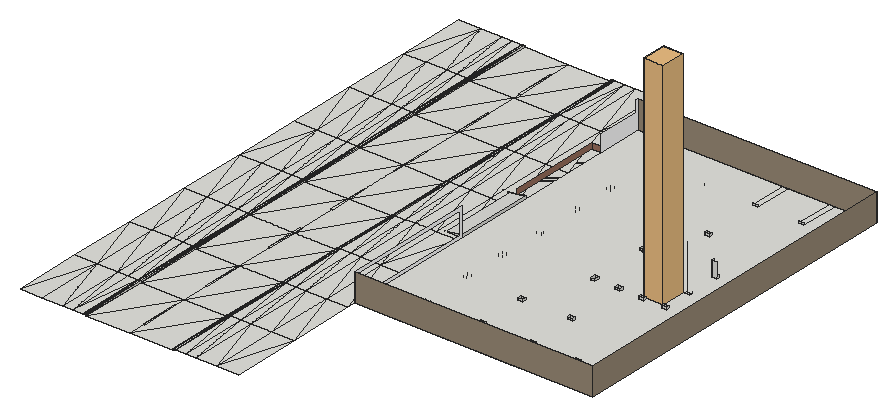
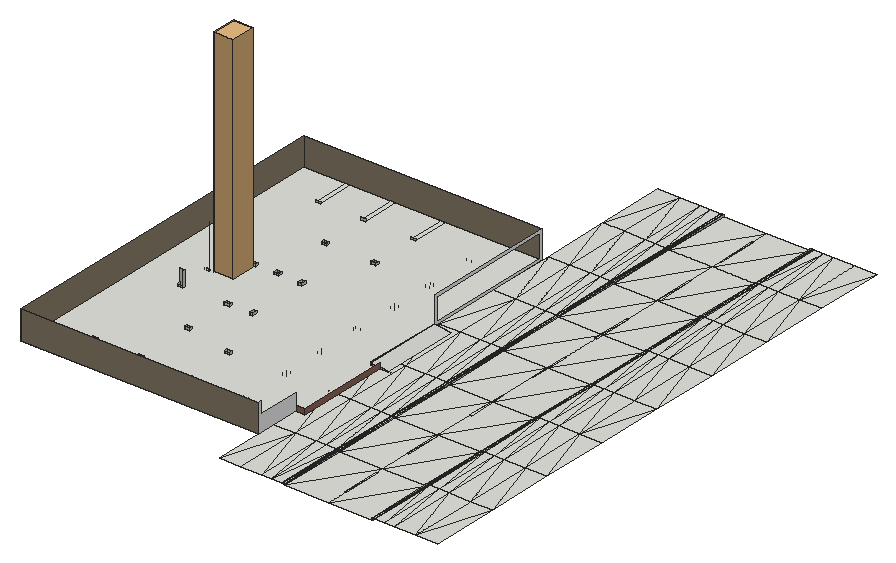
# SketchUp Ruby script. Lengths in inches.
U = 1.inch
M = Sketchup.active_model
def pt(a) = Geom::Point3d.new(a.map { |v| v * U })
def face(e, loops, mat)
  f = e.add_face(loops[0].map { |a| pt(a) })
  loops[1..].each { |l| e.add_face(l.map { |a| pt(a) }).erase! }
  f.material = f.back_material = mat if mat
  f
end
# faces: each face lists its corners as indices into pts; further lists are holes
def faces(e, pts, list, mat = nil) = list.each { |f| face(e, (f[0].is_a?(Array) ? f : [f]).map { |l| l.map { |i| pts[i] } }, mat) }
# xy, xz, yz: faces in a plane at the given z, y or x. An outline is a flat list of corners, or four numbers for a rectangle; further outlines are holes
def ring(l) = l.size == 4 ? [[l[0], l[1]], [l[2], l[1]], [l[2], l[3]], [l[0], l[3]]] : l.each_slice(2).to_a
def flat(e, list, mat, &to3) = list.each { |f| face(e, (f[0].is_a?(Array) ? f : [f]).map { |l| ring(l).map { |u, v| to3.(u, v) } }, mat) }
def xy(e, z, list, mat = nil) = flat(e, list, mat) { |x, y| [x, y, z] }
def xz(e, y, list, mat = nil) = flat(e, list, mat) { |x, z| [x, y, z] }
def yz(e, x, list, mat = nil) = flat(e, list, mat) { |y, z| [x, y, z] }
def lines(e, pts, list) = list.each { |a, b| e.add_line(pt(pts[a]), pt(pts[b])) }
# prism: a flat outline (further loops are holes) pulled along v
def prism(e, loops, v, mat = nil)
  f = face(e, loops, mat); d = Geom::Vector3d.new(v.map { |x| x * U })
  f.pushpull(f.normal.samedirection?(d) ? d.length : -d.length)
end
def box(e, o, s, mat = nil) = prism(e, [[o, [o[0] + s[0], o[1], o[2]], [o[0] + s[0], o[1] + s[1], o[2]], [o[0], o[1] + s[1], o[2]]]], [0, 0, s[2]], mat)
def at(x, y, z, deg = 0) = Geom::Transformation.translation(pt([x, y, z])) * Geom::Transformation.rotation(ORIGIN, Z_AXIS, deg.degrees)
def axes(o, x, y, z) = Geom::Transformation.new([*x, 0, *y, 0, *z, 0, *pt(o).to_a, 1])
def part(name) = M.definitions.add(name)
# library, detail: a bought-in or finely detailed component or shape, given as its bounding box
def library(name, o, s) = part(name).tap { |d| box(d.entities, o, s) }
def detail(e, o, s) = box(e.add_group.entities, o, s)
def put(e, d, t, mat = nil) = e.add_instance(d, t).tap { |i| i.material = mat if mat }
def group(e, t, mat = nil) = e.add_group.tap { |g| g.transformation = t; g.material = mat if mat }.entities
root = M.entities
M.materials.add("Bricks Weathered E01 100cm\#1").color = [154, 112, 93]
M.materials.add("Paint Brown Gloss 1.5cm").color = [255, 255, 255]
M.materials.add("Paint Brown Gloss 1.5cm\#1").color = [255, 255, 255]
M.materials.add("Wall Paint Bumpy 01 Ochre 100cm").color = [152, 138, 118]
c1 = library("Untitled",[11.72,11.72,0],[78.74,90.55,365.17])
xy(root,-10.11,[[1303.23,0,1424.89,0,1424.89,191.1],[1303.23,0,1424.89,191.1,1303.23,191.1],[1424.89,0,1546.54,0,1546.54,191.1],[1424.89,0,1546.54,191.1,1424.89,191.1],[1303.23,191.1,1424.89,191.1,1424.89,382.19],
  [1303.23,191.1,1424.89,382.19,1303.23,382.19],[1424.89,191.1,1546.54,191.1,1546.54,382.19],[1424.89,191.1,1546.54,382.19,1424.89,382.19],[1303.23,382.19,1424.89,382.19,1424.89,573.29],[1303.23,382.19,1424.89,573.29,1303.23,573.29],
  [1424.89,382.19,1546.54,382.19,1546.54,573.29],[1424.89,382.19,1546.54,573.29,1424.89,573.29],[1303.23,573.29,1424.89,573.29,1424.89,764.38],[1303.23,573.29,1424.89,764.38,1303.23,764.38],[1424.89,573.29,1546.54,573.29,1546.54,764.38],
  [1424.89,573.29,1546.54,764.38,1424.89,764.38],[1303.23,764.38,1424.89,764.38,1424.89,955.48],[1303.23,764.38,1424.89,955.48,1303.23,955.48],[1424.89,764.38,1546.54,764.38,1546.54,955.48],[1424.89,764.38,1546.54,955.48,1424.89,955.48],
  [1303.23,955.48,1424.89,1146.57,1303.23,1146.57],[1303.23,955.48,1424.89,955.48,1424.89,1146.57],[1424.89,955.48,1546.54,1146.57,1424.89,1146.57],[1424.89,955.48,1546.54,955.48,1546.54,1146.57],[1303.23,1146.57,1424.89,1146.57,1424.89,1337.67],
  [1303.23,1146.57,1424.89,1337.67,1303.23,1337.67],[1424.89,1146.57,1546.54,1146.57,1546.54,1337.67],[1424.89,1146.57,1546.54,1337.67,1424.89,1337.67],[1303.23,1337.67,1424.89,1337.67,1424.89,1528.76],[1303.23,1337.67,1424.89,1528.76,1303.23,1528.76],
  [1424.89,1337.67,1546.54,1337.67,1546.54,1528.76],[1424.89,1337.67,1546.54,1528.76,1424.89,1528.76]])
xy(root,-10.1,[[1422.83,51.125,1426.94,160.2,1422.83,160.2],[1422.83,51.125,1426.94,51.125,1426.94,160.2],[1422.83,269.27,1426.94,269.27,1426.94,378.35],[1422.83,269.27,1426.94,378.35,1422.83,378.35],[1422.83,487.42,1426.94,487.42,1426.94,596.5],
  [1422.83,487.42,1426.94,596.5,1422.83,596.5],[1422.83,705.57,1426.94,705.57,1426.94,814.64],[1422.83,705.57,1426.94,814.64,1422.83,814.64],[1422.83,923.72,1426.94,1032.79,1422.83,1032.79],[1422.83,923.72,1426.94,923.72,1426.94,1032.79],
  [1422.83,1141.87,1426.94,1141.87,1426.94,1250.94],[1422.83,1141.87,1426.94,1250.94,1422.83,1250.94],[1422.83,1360.02,1426.94,1360.02,1426.94,1469.09],[1422.83,1360.02,1426.94,1469.09,1422.83,1469.09]])
xy(root,-6,[[1296.67,0,1297.07,0,1297.07,0.65],[1296.67,0,1297.07,0.65,1296.67,0.65],[1297.07,0,1302.39,0,1302.39,0.65],[1297.07,0,1302.39,0.65,1297.07,0.65],[1302.39,0,1302.75,0,1302.75,0.65],
  [1302.39,0,1302.75,0.65,1302.39,0.65],[1547.03,0,1547.61,0,1547.61,0.61],[1547.03,0,1547.61,0.61,1547.03,0.61],[1547.61,0,1552.83,0,1552.83,0.61],[1547.61,0,1552.83,0.61,1547.61,0.61],
  [1552.83,0,1553.1,0,1553.1,0.61],[1552.83,0,1553.1,0.61,1552.83,0.61],[1553.68,0,1554.02,0,1554.02,191.1],[1553.68,0,1554.02,191.1,1553.68,191.1],[1554.02,0,1582.4375,0,1554.02,191.1],
  [1582.4375,0,1582.4375,191.1,1554.02,191.1],[1582.4375,0,1610.85,0,1582.4375,191.1],[1610.85,0,1610.85,191.1,1582.4375,191.1],[1610.85,0,1668.2,0,1610.85,191.1],[1668.2,0,1668.2,191.1,1610.85,191.1],
  [1668.2,0,1729.02,0,1729.02,191.09],[1668.2,0,1729.02,191.09,1668.2,191.1],[1120.75,0.01,1181.58,0.01,1181.58,191.1],[1120.75,0.01,1181.58,191.1,1120.75,191.1],[1181.58,0.01,1238.93,0.01,1181.58,191.1],
  [1238.93,0.01,1238.93,191.1,1181.58,191.1],[1238.93,0.01,1267.34,0.01,1238.93,191.1],[1267.34,0.01,1267.34,191.1,1238.93,191.1],[1267.34,0.01,1295.75,0.01,1295.75,191.1],[1267.34,0.01,1295.75,191.1,1267.34,191.1],
  [1295.75,0.01,1296.1,0.01,1296.1,191.1],[1295.75,0.01,1296.1,191.1,1295.75,191.1],[1547.03,0.61,1547.61,0.61,1547.61,191.1],[1547.03,0.61,1547.61,191.1,1547.03,191.1],[1547.61,0.61,1552.83,0.61,1552.83,191.1],
  [1547.61,0.61,1552.83,191.1,1547.61,191.1],[1552.83,0.61,1553.1,0.61,1553.1,191.1],[1552.83,0.61,1553.1,191.1,1552.83,191.1],[1296.67,0.65,1297.07,0.65,1297.07,191.1],[1296.67,0.65,1297.07,191.1,1296.67,191.1],
  [1297.07,0.65,1302.39,0.65,1302.39,191.1],[1297.07,0.65,1302.39,191.1,1297.07,191.1],[1302.39,0.65,1302.75,0.65,1302.75,191.1],[1302.39,0.65,1302.75,191.1,1302.39,191.1],[1729.02,191.09,1668.2,382.19,1668.2,191.1],
  [1729.02,191.09,1729.02,382.19,1668.2,382.19],[1120.75,191.1,1181.58,191.1,1120.75,382.2],[1181.58,191.1,1181.58,382.2,1120.75,382.2],[1181.58,191.1,1238.93,191.1,1181.58,382.2],[1238.93,191.1,1238.93,382.2,1181.58,382.2],
  [1238.93,191.1,1267.34,191.1,1238.93,382.2],[1267.34,191.1,1267.34,382.2,1238.93,382.2],[1267.34,191.1,1295.75,191.1,1267.34,382.2],[1295.75,191.1,1295.75,382.2,1267.34,382.2],[1295.75,191.1,1296.1,191.1,1296.1,382.2],
  [1295.75,191.1,1296.1,382.2,1295.75,382.2],[1296.67,191.1,1297.07,191.1,1297.07,382.19],[1296.67,191.1,1297.07,382.19,1296.67,382.19],[1297.07,191.1,1302.39,191.1,1297.07,382.19],[1302.39,191.1,1302.39,382.19,1297.07,382.19],
  [1302.39,191.1,1302.75,191.1,1302.39,382.19],[1302.75,191.1,1302.75,382.19,1302.39,382.19],[1547.03,191.1,1547.61,191.1,1547.61,382.19],[1547.03,191.1,1547.61,382.19,1547.03,382.19],[1547.61,191.1,1552.83,191.1,1547.61,382.19],
  [1552.83,191.1,1552.83,382.19,1547.61,382.19],[1552.83,191.1,1553.1,191.1,1552.83,382.19],[1553.1,191.1,1553.1,382.19,1552.83,382.19],[1553.68,191.1,1554.02,191.1,1554.02,382.19],[1553.68,191.1,1554.02,382.19,1553.68,382.19],
  [1554.02,191.1,1582.4375,191.1,1554.02,382.19],[1582.4375,191.1,1582.4375,382.19,1554.02,382.19],[1582.4375,191.1,1610.85,191.1,1582.4375,382.19],[1610.85,191.1,1610.85,382.19,1582.4375,382.19],[1610.85,191.1,1668.2,191.1,1610.85,382.19],
  [1668.2,191.1,1668.2,382.19,1610.85,382.19],[1296.67,382.19,1297.07,382.19,1297.07,573.29],[1296.67,382.19,1297.07,573.29,1296.67,573.29],[1297.07,382.19,1302.39,382.19,1297.07,573.29],[1302.39,382.19,1302.39,573.29,1297.07,573.29],
  [1302.39,382.19,1302.75,382.19,1302.39,573.29],[1302.75,382.19,1302.75,573.29,1302.39,573.29],[1547.03,382.19,1547.61,382.19,1547.61,573.29],[1547.03,382.19,1547.61,573.29,1547.03,573.29],[1547.61,382.19,1552.83,382.19,1547.61,573.29],
  [1552.83,382.19,1552.83,573.29,1547.61,573.29],[1552.83,382.19,1553.1,382.19,1552.83,573.29],[1553.1,382.19,1553.1,573.29,1552.83,573.29],[1553.68,382.19,1554.02,382.19,1554.02,573.29],[1553.68,382.19,1554.02,573.29,1553.68,573.29],
  [1554.02,382.19,1582.4375,382.19,1554.02,573.29],[1582.4375,382.19,1582.4375,573.29,1554.02,573.29],[1582.4375,382.19,1610.85,382.19,1582.4375,573.29],[1610.85,382.19,1610.85,573.29,1582.4375,573.29],[1610.85,382.19,1668.2,382.19,1610.85,573.29],
  [1668.2,382.19,1668.2,573.29,1610.85,573.29],[1668.2,382.19,1729.02,382.19,1668.2,573.29],[1729.02,382.19,1729.02,573.29,1668.2,573.29],[1120.75,382.2,1181.58,382.2,1120.75,573.29],[1181.58,382.2,1181.58,573.29,1120.75,573.29],
  [1181.58,382.2,1238.93,382.2,1181.58,573.29],[1238.93,382.2,1238.93,573.29,1181.58,573.29],[1238.93,382.2,1267.34,382.2,1238.93,573.29],[1267.34,382.2,1267.34,573.29,1238.93,573.29],[1267.34,382.2,1295.75,382.2,1267.34,573.29],
  [1295.75,382.2,1295.75,573.29,1267.34,573.29],[1295.75,382.2,1296.1,382.2,1296.1,573.29],[1295.75,382.2,1296.1,573.29,1295.75,573.29],[[1729.02,404.67,1729.02,1000.17,1704.32,1000.17,1704.32,1262.67,1729.02,1262.67,1729.02,1391.67,2132.52,1391.67,2132.52,1286.67,2146.52,1286.67,2146.52,1391.67,2262.52,1391.67,2262.52,1286.67,2276.52,1286.67,2276.52,1391.67,2393.52,1391.67,2393.52,404.67,2276.52,404.67,2276.52,509.67,2262.52,509.67,2262.52,404.67,2149.52,404.67,2149.52,509.67,2135.52,509.67,2135.52,404.67,2011.02,404.67,2011.02,509.67,1997.02,509.67,1997.02,404.67],[2132.52,980.67,2146.52,989.67],[2262.52,980.67,2276.52,989.67],[2262.52,806.67,2276.52,815.67],[2066.52,806.67,2075.52,820.67],[1997.02,1148.67,2011.02,1157.67],[2132.52,1118.67,2146.52,1127.67],[2066.52,975.67,2075.52,989.67],[2262.52,887.67,2276.52,896.67],[2132.52,806.67,2146.52,815.67],[1997.02,638.67,2011.02,647.67],[2198.52,806.67,2212.52,815.67],[2135.52,638.67,2149.52,647.67]],[1997.02,404.67,2011.02,509.67],
  [2135.52,404.67,2149.52,509.67],[2262.52,404.67,2276.52,509.67],[1120.75,573.29,1181.58,573.29,1120.75,764.39],[1181.58,573.29,1181.58,764.39,1120.75,764.39],[1181.58,573.29,1238.93,573.29,1181.58,764.39],
  [1238.93,573.29,1238.93,764.39,1181.58,764.39],[1238.93,573.29,1267.34,573.29,1238.93,764.39],[1267.34,573.29,1267.34,764.39,1238.93,764.39],[1267.34,573.29,1295.75,573.29,1267.34,764.39],[1295.75,573.29,1295.75,764.39,1267.34,764.39],
  [1295.75,573.29,1296.1,573.29,1296.1,764.39],[1295.75,573.29,1296.1,764.39,1295.75,764.39],[1296.67,573.29,1297.07,573.29,1296.67,764.38],[1297.07,573.29,1297.07,764.38,1296.67,764.38],[1297.07,573.29,1302.39,573.29,1297.07,764.38],
  [1302.39,573.29,1302.39,764.38,1297.07,764.38],[1302.39,573.29,1302.75,573.29,1302.75,764.38],[1302.39,573.29,1302.75,764.38,1302.39,764.38],[1547.03,573.29,1547.61,573.29,1547.03,764.38],[1547.61,573.29,1547.61,764.38,1547.03,764.38],
  [1547.61,573.29,1552.83,573.29,1547.61,764.38],[1552.83,573.29,1552.83,764.38,1547.61,764.38],[1552.83,573.29,1553.1,573.29,1553.1,764.38],[1552.83,573.29,1553.1,764.38,1552.83,764.38],[1553.68,573.29,1554.02,573.29,1553.68,764.38],
  [1554.02,573.29,1554.02,764.38,1553.68,764.38],[1554.02,573.29,1582.4375,573.29,1554.02,764.38],[1582.4375,573.29,1582.4375,764.38,1554.02,764.38],[1582.4375,573.29,1610.85,573.29,1582.4375,764.38],[1610.85,573.29,1610.85,764.38,1582.4375,764.38],
  [1610.85,573.29,1668.2,573.29,1610.85,764.38],[1668.2,573.29,1668.2,764.38,1610.85,764.38],[1668.2,573.29,1729.02,573.29,1729.02,764.38],[1668.2,573.29,1729.02,764.38,1668.2,764.38],[1997.02,638.67,2011.02,647.67],
  [2135.52,638.67,2149.52,647.67],[1296.67,764.38,1297.07,764.38,1297.07,955.48],[1296.67,764.38,1297.07,955.48,1296.67,955.48],[1297.07,764.38,1302.39,764.38,1297.07,955.48],[1302.39,764.38,1302.39,955.48,1297.07,955.48],
  [1302.39,764.38,1302.75,764.38,1302.39,955.48],[1302.75,764.38,1302.75,955.48,1302.39,955.48],[1547.03,764.38,1547.61,764.38,1547.61,955.48],[1547.03,764.38,1547.61,955.48,1547.03,955.48],[1547.61,764.38,1552.83,764.38,1547.61,955.48],
  [1552.83,764.38,1552.83,955.48,1547.61,955.48],[1552.83,764.38,1553.1,764.38,1552.83,955.48],[1553.1,764.38,1553.1,955.48,1552.83,955.48],[1553.68,764.38,1554.02,764.38,1554.02,955.48],[1553.68,764.38,1554.02,955.48,1553.68,955.48],
  [1554.02,764.38,1582.4375,764.38,1554.02,955.48],[1582.4375,764.38,1582.4375,955.48,1554.02,955.48],[1582.4375,764.38,1610.85,764.38,1582.4375,955.48],[1610.85,764.38,1610.85,955.48,1582.4375,955.48],[1610.85,764.38,1668.2,764.38,1610.85,955.48],
  [1668.2,764.38,1668.2,955.48,1610.85,955.48],[1668.2,764.38,1729.02,764.38,1668.2,955.48],[1729.02,764.38,1729.02,955.48,1668.2,955.48],[1120.75,764.39,1181.58,764.39,1181.58,955.48],[1120.75,764.39,1181.58,955.48,1120.75,955.48],
  [1181.58,764.39,1238.93,764.39,1181.58,955.48],[1238.93,764.39,1238.93,955.48,1181.58,955.48],[1238.93,764.39,1267.34,764.39,1238.93,955.48],[1267.34,764.39,1267.34,955.48,1238.93,955.48],[1267.34,764.39,1295.75,764.39,1267.34,955.48],
  [1295.75,764.39,1295.75,955.48,1267.34,955.48],[1295.75,764.39,1296.1,764.39,1295.75,955.48],[1296.1,764.39,1296.1,955.48,1295.75,955.48],[1709.42,778.97,1729.02,1000.17],[2066.52,806.67,2075.52,820.67],
  [2132.52,806.67,2146.52,815.67],[2198.52,806.67,2212.52,815.67],[2262.52,887.67,2276.52,896.67],[1120.75,955.48,1181.58,955.48,1120.75,1146.58],[1181.58,955.48,1181.58,1146.58,1120.75,1146.58],
  [1181.58,955.48,1238.93,955.48,1181.58,1146.58],[1238.93,955.48,1238.93,1146.58,1181.58,1146.58],[1238.93,955.48,1267.34,955.48,1238.93,1146.58],[1267.34,955.48,1267.34,1146.58,1238.93,1146.58],[1267.34,955.48,1295.75,955.48,1267.34,1146.58],
  [1295.75,955.48,1295.75,1146.58,1267.34,1146.58],[1295.75,955.48,1296.1,1146.58,1295.75,1146.58],[1295.75,955.48,1296.1,955.48,1296.1,1146.58],[1296.67,955.48,1297.07,1146.57,1296.67,1146.57],[1296.67,955.48,1297.07,955.48,1297.07,1146.57],
  [1297.07,955.48,1302.39,955.48,1297.07,1146.57],[1302.39,955.48,1302.39,1146.57,1297.07,1146.57],[1302.39,955.48,1302.75,955.48,1302.39,1146.57],[1302.75,955.48,1302.75,1146.57,1302.39,1146.57],[1547.03,955.48,1547.61,1146.57,1547.03,1146.57],
  [1547.03,955.48,1547.61,955.48,1547.61,1146.57],[1547.61,955.48,1552.83,955.48,1547.61,1146.57],[1552.83,955.48,1552.83,1146.57,1547.61,1146.57],[1552.83,955.48,1553.1,955.48,1552.83,1146.57],[1553.1,955.48,1553.1,1146.57,1552.83,1146.57],
  [1553.68,955.48,1554.02,1146.57,1553.68,1146.57],[1553.68,955.48,1554.02,955.48,1554.02,1146.57],[1554.02,955.48,1582.4375,955.48,1554.02,1146.57],[1582.4375,955.48,1582.4375,1146.57,1554.02,1146.57],[1582.4375,955.48,1610.85,955.48,1582.4375,1146.57],
  [1610.85,955.48,1610.85,1146.57,1582.4375,1146.57],[1610.85,955.48,1668.2,955.48,1610.85,1146.57],[1668.2,955.48,1668.2,1146.57,1610.85,1146.57],[1668.2,955.48,1729.02,955.48,1668.2,1146.57],[1729.02,955.48,1729.02,1146.57,1668.2,1146.57],
  [2066.52,975.67,2075.52,989.67],[2132.52,980.67,2146.52,989.67],[2262.52,980.67,2276.52,989.67],[2132.52,1118.67,2146.52,1127.67],[1296.67,1146.57,1297.07,1146.57,1297.07,1337.67],
  [1296.67,1146.57,1297.07,1337.67,1296.67,1337.67],[1297.07,1146.57,1302.39,1146.57,1297.07,1337.67],[1302.39,1146.57,1302.39,1337.67,1297.07,1337.67],[1302.39,1146.57,1302.75,1146.57,1302.39,1337.67],[1302.75,1146.57,1302.75,1337.67,1302.39,1337.67],
  [1547.03,1146.57,1547.61,1146.57,1547.61,1337.67],[1547.03,1146.57,1547.61,1337.67,1547.03,1337.67],[1547.61,1146.57,1552.83,1146.57,1547.61,1337.67],[1552.83,1146.57,1552.83,1337.67,1547.61,1337.67],[1552.83,1146.57,1553.1,1146.57,1552.83,1337.67],
  [1553.1,1146.57,1553.1,1337.67,1552.83,1337.67],[1553.68,1146.57,1554.02,1146.57,1554.02,1337.67],[1553.68,1146.57,1554.02,1337.67,1553.68,1337.67],[1554.02,1146.57,1582.4375,1146.57,1554.02,1337.67],[1582.4375,1146.57,1582.4375,1337.67,1554.02,1337.67],
  [1582.4375,1146.57,1610.85,1146.57,1582.4375,1337.67],[1610.85,1146.57,1610.85,1337.67,1582.4375,1337.67],[1610.85,1146.57,1668.2,1146.57,1610.85,1337.67],[1668.2,1146.57,1668.2,1337.67,1610.85,1337.67],[1668.2,1146.57,1729.02,1146.57,1668.2,1337.67],
  [1729.02,1146.57,1729.02,1337.67,1668.2,1337.67],[1120.75,1146.58,1181.58,1146.58,1120.75,1337.67],[1181.58,1146.58,1181.58,1337.67,1120.75,1337.67],[1181.58,1146.58,1238.93,1146.58,1181.58,1337.67],[1238.93,1146.58,1238.93,1337.67,1181.58,1337.67],
  [1238.93,1146.58,1267.34,1146.58,1238.93,1337.67],[1267.34,1146.58,1267.34,1337.67,1238.93,1337.67],[1267.34,1146.58,1295.75,1146.58,1267.34,1337.67],[1295.75,1146.58,1295.75,1337.67,1267.34,1337.67],[1295.75,1146.58,1296.1,1146.58,1296.1,1337.67],
  [1295.75,1146.58,1296.1,1337.67,1295.75,1337.67],[1997.02,1148.67,2011.02,1157.67],[2132.52,1286.67,2146.52,1391.67],[2262.52,1286.67,2276.52,1391.67],[1120.75,1337.67,1181.58,1337.67,1181.58,1528.77],
  [1120.75,1337.67,1181.58,1528.77,1120.75,1528.77],[1181.58,1337.67,1238.93,1337.67,1181.58,1528.77],[1238.93,1337.67,1238.93,1528.77,1181.58,1528.77],[1238.93,1337.67,1267.34,1337.67,1238.93,1528.77],[1267.34,1337.67,1267.34,1528.77,1238.93,1528.77],
  [1267.34,1337.67,1295.75,1337.67,1267.34,1528.77],[1295.75,1337.67,1295.75,1528.77,1267.34,1528.77],[1295.75,1337.67,1296.1,1337.67,1296.1,1528.77],[1295.75,1337.67,1296.1,1528.77,1295.75,1528.77],[1296.67,1337.67,1297.07,1337.67,1297.07,1527.99],
  [1296.67,1337.67,1297.07,1527.99,1296.67,1527.99],[1297.07,1337.67,1302.39,1337.67,1302.39,1527.99],[1297.07,1337.67,1302.39,1527.99,1297.07,1527.99],[1302.39,1337.67,1302.75,1337.67,1302.75,1527.99],[1302.39,1337.67,1302.75,1527.99,1302.39,1527.99],
  [1547.03,1337.67,1547.61,1337.67,1547.61,1528.125],[1547.03,1337.67,1547.61,1528.125,1547.03,1528.125],[1547.61,1337.67,1552.83,1337.67,1552.83,1528.125],[1547.61,1337.67,1552.83,1528.125,1547.61,1528.125],[1552.83,1337.67,1553.1,1337.67,1553.1,1528.125],
  [1552.83,1337.67,1553.1,1528.125,1552.83,1528.125],[1553.68,1337.67,1554.02,1337.67,1554.02,1528.76],[1553.68,1337.67,1554.02,1528.76,1553.68,1528.76],[1554.02,1337.67,1582.4375,1337.67,1582.4375,1528.76],[1554.02,1337.67,1582.4375,1528.76,1554.02,1528.76],
  [1582.4375,1337.67,1610.85,1337.67,1582.4375,1528.76],[1610.85,1337.67,1610.85,1528.76,1582.4375,1528.76],[1610.85,1337.67,1668.2,1337.67,1610.85,1528.76],[1668.2,1337.67,1668.2,1528.76,1610.85,1528.76],[1668.2,1337.67,1729.02,1337.67,1729.02,1528.76],
  [1668.2,1337.67,1729.02,1528.76,1668.2,1528.76],[1296.67,1527.99,1297.07,1527.99,1297.07,1528.76],[1296.67,1527.99,1297.07,1528.76,1296.67,1528.76],[1297.07,1527.99,1302.39,1527.99,1302.39,1528.76],[1297.07,1527.99,1302.39,1528.76,1297.07,1528.76],
  [1302.39,1527.99,1302.75,1527.99,1302.75,1528.76],[1302.39,1527.99,1302.75,1528.76,1302.39,1528.76],[1547.03,1528.125,1547.61,1528.125,1547.61,1528.76],[1547.03,1528.125,1547.61,1528.76,1547.03,1528.76],[1547.61,1528.125,1552.83,1528.125,1552.83,1528.76],
  [1547.61,1528.125,1552.83,1528.76,1547.61,1528.76],[1552.83,1528.125,1553.1,1528.125,1553.1,1528.76],[1552.83,1528.125,1553.1,1528.76,1552.83,1528.76]])
xz(root,404.67,[[1729.02,-6,2393.52,72]],"Wall Paint Bumpy 01 Ochre 100cm")
xz(root,509.67,[[1997.02,-6,2011.02,0],[2135.52,-6,2149.52,0],[2262.52,-6,2276.52,0]])
xz(root,638.67,[[1997.02,-6,2011.02,0],[2135.52,-6,2149.52,0]])
xz(root,647.67,[[1997.02,-6,2011.02,0],[2135.52,-6,2149.52,0]])
xz(root,778.97,[[1659.27,-9.61,1709.42,-6,1729.02,-6,1729.02,0.9]])
xz(root,806.67,[[2066.52,-6,2075.52,0],[2132.52,-6,2146.52,0],[2198.52,-6,2212.52,0],[2262.52,-6,2276.52,0]])
xz(root,815.67,[[2132.52,-6,2146.52,0],[2198.52,-6,2212.52,0],[2262.52,-6,2276.52,0]])
xz(root,820.67,[[2066.52,-6,2075.52,0]])
xz(root,975.67,[[2066.52,-6,2075.52,0]])
xz(root,980.67,[[2132.52,-6,2146.52,0],[2262.52,-6,2276.52,36]])
xz(root,989.67,[[2066.52,-6,2075.52,0],[2132.52,-6,2146.52,0],[2262.52,-6,2276.52,0]])
xz(root,1000.17,[[1659.27,-9.61,1704.32,-2.82,1704.32,-6,1709.42,-6],[1704.32,-6,1704.32,-2.82,1723.05,0,1729.02,0,1729.02,-6]])
xz(root,1118.67,[[2132.52,-6,2146.52,0]])
xz(root,1127.67,[[2132.52,-6,2146.52,0]])
xz(root,1148.67,[[1997.02,-6,2011.02,0]])
xz(root,1157.67,[[1997.02,-6,2011.02,0]])
xz(root,1262.67,[[1704.32,-6,1729.02,9.5]],"Bricks Weathered E01 100cm\#1")
xz(root,1286.67,[[2132.52,-6,2146.52,0],[2262.52,-6,2276.52,0]])
xz(root,1391.67,[[1729.02,-6,2393.52,72]],"Wall Paint Bumpy 01 Ochre 100cm")
yz(root,1296.31,[[0.01,-6.69,191.1,-6.69,0.01,-6.26],[191.1,-6.69,191.1,-6.26,0.01,-6.26],[191.1,-6.69,382.2,-6.26,191.1,-6.26],[191.1,-6.69,382.2,-6.69,382.2,-6.26],[382.2,-6.69,573.29,-6.26,382.2,-6.26],
  [382.2,-6.69,573.29,-6.69,573.29,-6.26],[573.29,-6.69,764.39,-6.26,573.29,-6.26],[573.29,-6.69,764.39,-6.69,764.39,-6.26],[764.39,-6.69,955.48,-6.26,764.39,-6.26],[764.39,-6.69,955.48,-6.69,955.48,-6.26],
  [955.48,-6.69,1146.58,-6.26,955.48,-6.26],[955.48,-6.69,1146.58,-6.69,1146.58,-6.26],[1146.58,-6.69,1337.67,-6.26,1146.58,-6.26],[1146.58,-6.69,1337.67,-6.69,1337.67,-6.26],[1337.67,-6.69,1528.77,-6.69,1337.67,-6.26],
  [1528.77,-6.69,1528.77,-6.26,1337.67,-6.26]])
yz(root,1296.46,[[0,-6.75,0,-6.26,0.65,-6.26],[0,-6.75,0.65,-6.26,0.65,-6.75],[0.65,-6.75,0.65,-6.26,191.1,-6.26],[0.65,-6.75,191.1,-6.26,191.1,-6.75],[191.1,-6.75,191.1,-6.26,382.19,-6.75],
  [382.19,-6.75,191.1,-6.26,382.19,-6.26],[382.19,-6.75,382.19,-6.26,573.29,-6.75],[573.29,-6.75,382.19,-6.26,573.29,-6.26],[573.29,-6.75,573.29,-6.26,764.38,-6.75],[764.38,-6.75,573.29,-6.26,764.38,-6.26],
  [764.38,-6.75,764.38,-6.26,955.48,-6.75],[955.48,-6.75,764.38,-6.26,955.48,-6.26],[1146.57,-6.75,955.48,-6.26,1146.57,-6.26],[955.48,-6.75,955.48,-6.26,1146.57,-6.75],[1146.57,-6.75,1146.57,-6.26,1337.67,-6.75],
  [1337.67,-6.75,1146.57,-6.26,1337.67,-6.26],[1337.67,-6.75,1337.67,-6.26,1527.99,-6.26],[1337.67,-6.75,1527.99,-6.26,1527.99,-6.75],[1527.99,-6.75,1527.99,-6.26,1528.76,-6.26],[1527.99,-6.75,1528.76,-6.26,1528.76,-6.75]])
yz(root,1303.23,[[0,-10.11,0.65,-10.11,0,-7.1875],[0.65,-10.11,0.65,-7.1875,0,-7.1875],[0.65,-10.11,191.1,-10.11,0.65,-7.1875],[191.1,-10.11,191.1,-7.1875,0.65,-7.1875],[191.1,-10.11,382.19,-10.11,382.19,-7.1875],
  [191.1,-10.11,382.19,-7.1875,191.1,-7.1875],[382.19,-10.11,573.29,-10.11,573.29,-7.1875],[382.19,-10.11,573.29,-7.1875,382.19,-7.1875],[573.29,-10.11,764.38,-10.11,573.29,-7.1875],[764.38,-10.11,764.38,-7.1875,573.29,-7.1875],
  [764.38,-10.11,955.48,-10.11,955.48,-7.1875],[764.38,-10.11,955.48,-7.1875,764.38,-7.1875],[955.48,-10.11,1146.57,-10.11,1146.57,-7.1875],[955.48,-10.11,1146.57,-7.1875,955.48,-7.1875],[1146.57,-10.11,1337.67,-10.11,1337.67,-7.1875],
  [1146.57,-10.11,1337.67,-7.1875,1146.57,-7.1875],[1337.67,-10.11,1527.99,-10.11,1337.67,-7.1875],[1527.99,-10.11,1527.99,-7.1875,1337.67,-7.1875],[1527.99,-10.11,1528.76,-10.11,1527.99,-7.1875],[1528.76,-10.11,1528.76,-7.1875,1527.99,-7.1875],
  [0,-7.1875,0.65,-7.1875,0,-6.49],[0.65,-7.1875,0.65,-6.49,0,-6.49],[0.65,-7.1875,191.1,-7.1875,0.65,-6.49],[191.1,-7.1875,191.1,-6.49,0.65,-6.49],[191.1,-7.1875,382.19,-7.1875,191.1,-6.49],
  [382.19,-7.1875,382.19,-6.49,191.1,-6.49],[382.19,-7.1875,573.29,-7.1875,382.19,-6.49],[573.29,-7.1875,573.29,-6.49,382.19,-6.49],[573.29,-7.1875,764.38,-6.49,573.29,-6.49],[573.29,-7.1875,764.38,-7.1875,764.38,-6.49],
  [764.38,-7.1875,955.48,-7.1875,764.38,-6.49],[955.48,-7.1875,955.48,-6.49,764.38,-6.49],[1146.57,-7.1875,1146.57,-6.49,955.48,-6.49],[955.48,-7.1875,1146.57,-7.1875,955.48,-6.49],[1146.57,-7.1875,1337.67,-7.1875,1146.57,-6.49],
  [1337.67,-7.1875,1337.67,-6.49,1146.57,-6.49],[1337.67,-7.1875,1527.99,-7.1875,1337.67,-6.49],[1527.99,-7.1875,1527.99,-6.49,1337.67,-6.49],[1527.99,-7.1875,1528.76,-7.1875,1527.99,-6.49],[1528.76,-7.1875,1528.76,-6.49,1527.99,-6.49]])
yz(root,1546.54,[[0,-10.11,0,-6.93,0.61,-6.93],[0,-10.11,0.61,-6.93,0.61,-10.11],[0.61,-10.11,0.61,-6.93,191.1,-6.93],[0.61,-10.11,191.1,-6.93,191.1,-10.11],[191.1,-10.11,191.1,-6.93,382.19,-6.93],
  [191.1,-10.11,382.19,-6.93,382.19,-10.11],[382.19,-10.11,382.19,-6.93,573.29,-6.93],[382.19,-10.11,573.29,-6.93,573.29,-10.11],[573.29,-10.11,573.29,-6.93,764.38,-10.11],[764.38,-10.11,573.29,-6.93,764.38,-6.93],
  [764.38,-10.11,764.38,-6.93,955.48,-6.93],[764.38,-10.11,955.48,-6.93,955.48,-10.11],[955.48,-10.11,1146.57,-6.93,1146.57,-10.11],[955.48,-10.11,955.48,-6.93,1146.57,-6.93],[1146.57,-10.11,1146.57,-6.93,1337.67,-6.93],
  [1146.57,-10.11,1337.67,-6.93,1337.67,-10.11],[1337.67,-10.11,1337.67,-6.93,1528.125,-6.93],[1337.67,-10.11,1528.125,-6.93,1528.125,-10.11],[1528.125,-10.11,1528.125,-6.93,1528.76,-6.93],[1528.125,-10.11,1528.76,-6.93,1528.76,-10.11],
  [0,-6.93,0,-6.49,0.61,-6.49],[0,-6.93,0.61,-6.49,0.61,-6.93],[0.61,-6.93,0.61,-6.49,191.1,-6.49],[0.61,-6.93,191.1,-6.49,191.1,-6.93],[191.1,-6.93,191.1,-6.49,382.19,-6.93],
  [382.19,-6.93,191.1,-6.49,382.19,-6.49],[382.19,-6.93,382.19,-6.49,573.29,-6.93],[573.29,-6.93,382.19,-6.49,573.29,-6.49],[573.29,-6.93,573.29,-6.49,764.38,-6.49],[573.29,-6.93,764.38,-6.49,764.38,-6.93],
  [764.38,-6.93,764.38,-6.49,955.48,-6.93],[955.48,-6.93,764.38,-6.49,955.48,-6.49],[1146.57,-6.93,955.48,-6.49,1146.57,-6.49],[955.48,-6.93,955.48,-6.49,1146.57,-6.93],[1146.57,-6.93,1146.57,-6.49,1337.67,-6.93],
  [1337.67,-6.93,1146.57,-6.49,1337.67,-6.49],[1337.67,-6.93,1337.67,-6.49,1528.125,-6.49],[1337.67,-6.93,1528.125,-6.49,1528.125,-6.93],[1528.125,-6.93,1528.125,-6.49,1528.76,-6.49],[1528.125,-6.93,1528.76,-6.49,1528.76,-6.93]])
yz(root,1553.31,[[0,-6.69,0.61,-6.69,0,-6.26],[0.61,-6.69,0.61,-6.26,0,-6.26],[0.61,-6.69,191.1,-6.69,0.61,-6.26],[191.1,-6.69,191.1,-6.26,0.61,-6.26],[191.1,-6.69,382.19,-6.26,191.1,-6.26],
  [191.1,-6.69,382.19,-6.69,382.19,-6.26],[382.19,-6.69,573.29,-6.26,382.19,-6.26],[382.19,-6.69,573.29,-6.69,573.29,-6.26],[573.29,-6.69,764.38,-6.26,573.29,-6.26],[573.29,-6.69,764.38,-6.69,764.38,-6.26],
  [764.38,-6.69,955.48,-6.26,764.38,-6.26],[764.38,-6.69,955.48,-6.69,955.48,-6.26],[955.48,-6.69,1146.57,-6.26,955.48,-6.26],[955.48,-6.69,1146.57,-6.69,1146.57,-6.26],[1146.57,-6.69,1337.67,-6.26,1146.57,-6.26],
  [1146.57,-6.69,1337.67,-6.69,1337.67,-6.26],[1337.67,-6.69,1528.125,-6.69,1337.67,-6.26],[1528.125,-6.69,1528.125,-6.26,1337.67,-6.26],[1528.125,-6.69,1528.76,-6.69,1528.125,-6.26],[1528.76,-6.69,1528.76,-6.26,1528.125,-6.26]])
yz(root,1553.47,[[0,-6.69,0,-6.26,191.1,-6.26],[0,-6.69,191.1,-6.26,191.1,-6.69],[191.1,-6.69,191.1,-6.26,382.19,-6.69],[382.19,-6.69,191.1,-6.26,382.19,-6.26],[382.19,-6.69,382.19,-6.26,573.29,-6.69],
  [573.29,-6.69,382.19,-6.26,573.29,-6.26],[573.29,-6.69,573.29,-6.26,764.38,-6.69],[764.38,-6.69,573.29,-6.26,764.38,-6.26],[764.38,-6.69,764.38,-6.26,955.48,-6.69],[955.48,-6.69,764.38,-6.26,955.48,-6.26],
  [1146.57,-6.69,955.48,-6.26,1146.57,-6.26],[955.48,-6.69,955.48,-6.26,1146.57,-6.69],[1146.57,-6.69,1146.57,-6.26,1337.67,-6.69],[1337.67,-6.69,1146.57,-6.26,1337.67,-6.26],[1337.67,-6.69,1337.67,-6.26,1528.76,-6.26],
  [1337.67,-6.69,1528.76,-6.26,1528.76,-6.69]])
yz(root,1704.32,[[1000.17,-6,1000.17,0,1001.07,0,1001.07,9.5,1262.67,9.5,1262.67,-6]],"Bricks Weathered E01 100cm\#1")
yz(root,1729.02,[[778.17,-6,778.97,0],[778.97,-6,1000.17,0]])
yz(root,1729.02,[[1262.67,-6,1262.67,40.2,1382.67,40.2,1382.67,72,1391.67,72,1391.67,-6]],"Paint Brown Gloss 1.5cm")
yz(root,1729.02,[[[404.67,-6,778.17,72],[411.88,1.21,770.97,64.79]]],"Paint Brown Gloss 1.5cm\#1")
yz(root,1997.02,[[638.67,-6,647.67,0],[1148.67,-6,1157.67,0]])
yz(root,2011.02,[[638.67,-6,647.67,0],[1148.67,-6,1157.67,0]])
yz(root,2066.52,[[806.67,-6,820.67,0],[975.67,-6,989.67,0]])
yz(root,2075.52,[[806.67,-6,820.67,0],[975.67,-6,989.67,0]])
yz(root,2132.52,[[806.67,-6,815.67,0],[980.67,-6,989.67,0],[1118.67,-6,1127.67,0]])
yz(root,2135.52,[[638.67,-6,647.67,0]])
yz(root,2146.52,[[806.67,-6,815.67,0],[980.67,-6,989.67,0],[1118.67,-6,1127.67,0]])
yz(root,2149.52,[[638.67,-6,647.67,0]])
yz(root,2198.52,[[806.67,-6,815.67,0]])
yz(root,2212.52,[[806.67,-6,815.67,0]])
yz(root,2262.52,[[806.67,-6,815.67,0],[980.67,-6,989.67,36]])
yz(root,2276.52,[[806.67,-6,815.67,0],[980.67,-6,989.67,0]])
yz(root,2393.52,[[404.67,-6,1391.67,72]],"Wall Paint Bumpy 01 Ochre 100cm")
p = [[1704.32,1000.17,-2.82],[1659.27,1000.17,-9.61],[1659.27,778.97,-9.61],[1729.02,778.97,0.9],[1729.02,1000.17,0.9],[1723.05,1000.17,0],
  [1709.42,1000.17,-6],[1709.42,778.97,-6],[1303.23,0.65,-6.49],[1303.11,0.65,-6.12],[1303.11,0,-6.12],[1303.23,0,-6.49],
  [1546.54,0,-6.49],[1546.66,0,-6.125],[1546.66,0.61,-6.125],[1546.54,0.61,-6.49],[1546.54,191.1,-6.49],[1546.66,191.1,-6.125],
  [1303.23,191.1,-6.49],[1303.11,191.1,-6.12],[1303.23,382.19,-6.49],[1303.11,382.19,-6.12],[1546.66,382.19,-6.125],[1546.54,382.19,-6.49],
  [1303.23,573.29,-6.49],[1303.11,573.29,-6.12],[1546.66,573.29,-6.125],[1546.54,573.29,-6.49],[1303.23,764.38,-6.49],[1303.11,764.38,-6.12],
  [1546.66,764.38,-6.125],[1546.54,764.38,-6.49],[1303.23,955.48,-6.49],[1303.11,955.48,-6.12],[1546.66,955.48,-6.125],[1546.54,955.48,-6.49],
  [1303.23,1146.57,-6.49],[1303.11,1146.57,-6.12],[1546.66,1146.57,-6.125],[1546.54,1146.57,-6.49],[1303.23,1337.67,-6.49],[1303.11,1337.67,-6.12],
  [1546.66,1337.67,-6.125],[1546.54,1337.67,-6.49],[1303.23,1527.99,-6.49],[1303.11,1527.99,-6.12],[1546.66,1528.125,-6.125],[1546.54,1528.125,-6.49],
  [1303.23,1528.76,-6.49],[1303.11,1528.76,-6.12],[1546.66,1528.76,-6.125],[1546.54,1528.76,-6.49],[1296.1,0.01,-6],[1296.31,0.01,-6.26],
  [1296.31,191.1,-6.26],[1296.1,191.1,-6],[1296.67,0.65,-6],[1296.46,0.65,-6.26],[1296.46,0,-6.26],[1296.67,0,-6],
  [1553.31,0.61,-6.26],[1553.1,0.61,-6],[1553.1,0,-6],[1553.31,0,-6.26],[1553.68,191.1,-6],[1553.47,191.1,-6.26],
  [1553.47,0,-6.26],[1553.68,0,-6],[1553.31,191.1,-6.26],[1553.1,191.1,-6],[1296.67,191.1,-6],[1296.46,191.1,-6.26],
  [1296.31,382.2,-6.26],[1296.1,382.2,-6],[1296.67,382.19,-6],[1296.46,382.19,-6.26],[1553.31,382.19,-6.26],[1553.1,382.19,-6],
  [1553.68,382.19,-6],[1553.47,382.19,-6.26],[1296.31,573.29,-6.26],[1296.1,573.29,-6],[1296.67,573.29,-6],[1296.46,573.29,-6.26],
  [1553.31,573.29,-6.26],[1553.1,573.29,-6],[1553.68,573.29,-6],[1553.47,573.29,-6.26],[1296.31,764.39,-6.26],[1296.1,764.39,-6],
  [1296.67,764.38,-6],[1296.46,764.38,-6.26],[1553.31,764.38,-6.26],[1553.1,764.38,-6],[1553.68,764.38,-6],[1553.47,764.38,-6.26],
  [1296.31,955.48,-6.26],[1296.1,955.48,-6],[1296.67,955.48,-6],[1296.46,955.48,-6.26],[1553.31,955.48,-6.26],[1553.1,955.48,-6],
  [1553.68,955.48,-6],[1553.47,955.48,-6.26],[1296.31,1146.58,-6.26],[1296.1,1146.58,-6],[1296.67,1146.57,-6],[1296.46,1146.57,-6.26],
  [1553.31,1146.57,-6.26],[1553.1,1146.57,-6],[1553.68,1146.57,-6],[1553.47,1146.57,-6.26],[1296.31,1337.67,-6.26],[1296.1,1337.67,-6],
  [1296.67,1337.67,-6],[1296.46,1337.67,-6.26],[1553.31,1337.67,-6.26],[1553.1,1337.67,-6],[1553.68,1337.67,-6],[1553.47,1337.67,-6.26],
  [1296.31,1528.77,-6.26],[1296.1,1528.77,-6],[1296.67,1527.99,-6],[1296.46,1527.99,-6.26],[1553.31,1528.125,-6.26],[1553.1,1528.125,-6],
  [1553.68,1528.76,-6],[1553.47,1528.76,-6.26],[1296.67,1528.76,-6],[1296.46,1528.76,-6.26],[1553.31,1528.76,-6.26],[1553.1,1528.76,-6],
  [1302.75,0.65,-6],[1302.75,0,-6],[1547.03,0,-6],[1547.03,0.61,-6],[1547.03,191.1,-6],[1302.75,191.1,-6],
  [1302.75,382.19,-6],[1547.03,382.19,-6],[1302.75,573.29,-6],[1547.03,573.29,-6],[1302.75,764.38,-6],[1547.03,764.38,-6],
  [1302.75,955.48,-6],[1547.03,955.48,-6],[1302.75,1146.57,-6],[1547.03,1146.57,-6],[1302.75,1337.67,-6],[1547.03,1337.67,-6],
  [1302.75,1527.99,-6],[1547.03,1528.125,-6],[1302.75,1528.76,-6],[1547.03,1528.76,-6],[2276.52,896.67,0],[2276.52,896.67,-6],
  [2262.52,896.67,-6],[2262.52,896.67,120],[1843.02,641.67,0],[1843.02,641.67,-6],[1852.02,1154.67,0],[1852.02,1154.67,-6],
  [1997.02,1286.67,0],[1997.02,1286.67,-6],[1843.02,1154.67,0],[1843.02,1154.67,-6],[1843.02,777.67,0],[1843.02,777.67,-6],
  [1852.02,1018.67,0],[1852.02,1018.67,-6],[1843.02,509.67,0],[1843.02,509.67,-6],[1852.02,1140.67,0],[1852.02,1140.67,-6],
  [1857.02,1286.67,0],[1857.02,1286.67,-6],[1852.02,777.67,0],[1852.02,777.67,-6],[1852.02,1032.67,0],[1852.02,1032.67,-6],
  [1843.02,763.67,0],[1843.02,763.67,-6],[1852.02,655.67,0],[1852.02,655.67,-6],[1857.02,509.67,0],[1857.02,509.67,-6],
  [1852.02,763.67,0],[1852.02,763.67,-6],[1843.02,1032.67,0],[1843.02,1032.67,-6],[1843.02,1286.67,0],[1843.02,1286.67,-6],
  [1852.02,641.67,0],[1852.02,641.67,-6],[1843.02,1140.67,0],[1843.02,1140.67,-6],[1843.02,655.67,0],[1843.02,655.67,-6],
  [1843.02,893.67,0],[1843.02,893.67,-6],[1857.02,893.67,0],[1857.02,893.67,-6],[1857.02,902.67,0],[1857.02,902.67,-6]]
faces(root,p,[[0,1,2,3,4,5],[6,7,2,1],[8,9,10],[10,11,8],[12,13,14],[14,15,12],[16,15,14],[14,17,16],
  [18,19,9],[9,8,18],[20,21,19],[19,18,20],[16,17,22],[22,23,16],[24,25,21],[21,20,24],
  [26,27,23],[23,22,26],[28,29,25],[25,24,28],[27,26,30],[30,31,27],[32,33,29],[29,28,32],
  [31,30,34],[34,35,31],[36,37,33],[33,32,36],[35,34,38],[38,39,35],[40,41,37],[37,36,40],
  [42,43,39],[39,38,42],[40,44,45],[45,41,40],[43,42,46],[46,47,43],[48,49,45],[45,44,48],
  [47,46,50],[50,51,47],[52,53,54],[54,55,52],[56,57,58],[58,59,56],[60,61,62],[62,63,60],
  [64,65,66],[66,67,64],[68,69,61],[61,60,68],[70,71,57],[57,56,70],[55,54,72],[72,73,55],
  [74,75,71],[71,70,74],[69,68,76],[76,77,69],[65,64,78],[78,79,65],[73,72,80],[80,81,73],
  [82,83,75],[75,74,82],[77,76,84],[84,85,77],[86,87,79],[79,78,86],[81,80,88],[88,89,81],
  [90,91,83],[83,82,90],[85,84,92],[92,93,85],[87,86,94],[94,95,87],[89,88,96],[96,97,89],
  [98,99,91],[91,90,98],[93,92,100],[100,101,93],[102,103,95],[95,94,102],[97,96,104],[104,105,97],
  [106,107,99],[99,98,106],[101,100,108],[108,109,101],[103,102,110],[110,111,103],[105,104,112],[112,113,105],
  [114,115,107],[107,106,114],[109,108,116],[116,117,109],[118,119,111],[111,110,118],[113,112,120],[120,121,113],
  [122,123,115],[115,114,122],[116,124,125],[125,117,116],[126,127,119],[119,118,126],[123,122,128],[128,129,123],
  [130,131,125],[125,124,130],[9,132,133],[133,10,9],[13,134,135],[135,14,13],[17,14,135],[135,136,17],
  [19,137,132],[132,9,19],[21,138,137],[137,19,21],[17,136,139],[139,22,17],[25,140,138],[138,21,25],
  [141,26,22],[22,139,141],[140,25,29],[29,142,140],[26,141,143],[143,30,26],[33,144,142],[142,29,33],
  [30,143,145],[145,34,30],[37,146,144],[144,33,37],[34,145,147],[147,38,34],[41,148,146],[146,37,41],
  [149,42,38],[38,147,149],[41,45,150],[150,148,41],[42,149,151],[151,46,42],[49,152,150],[150,45,49],
  [46,151,153],[153,50,46]])
lines(root,p,[[154,155],[156,157],[158,159],[160,161],[162,163],[164,165],[166,167],[168,169],[170,171],[172,173],[174,175],[176,177],
  [178,179],[180,181],[182,183],[184,185],[186,187],[188,189],[190,191],[192,193],[194,195],[196,197],[198,199],[200,201],
  [202,203]])
put(root,c1,axes([2263.36,809.55,-81.27],[0,0.8636,0],[-0.59,0,0],[0,0,1.84008]))
